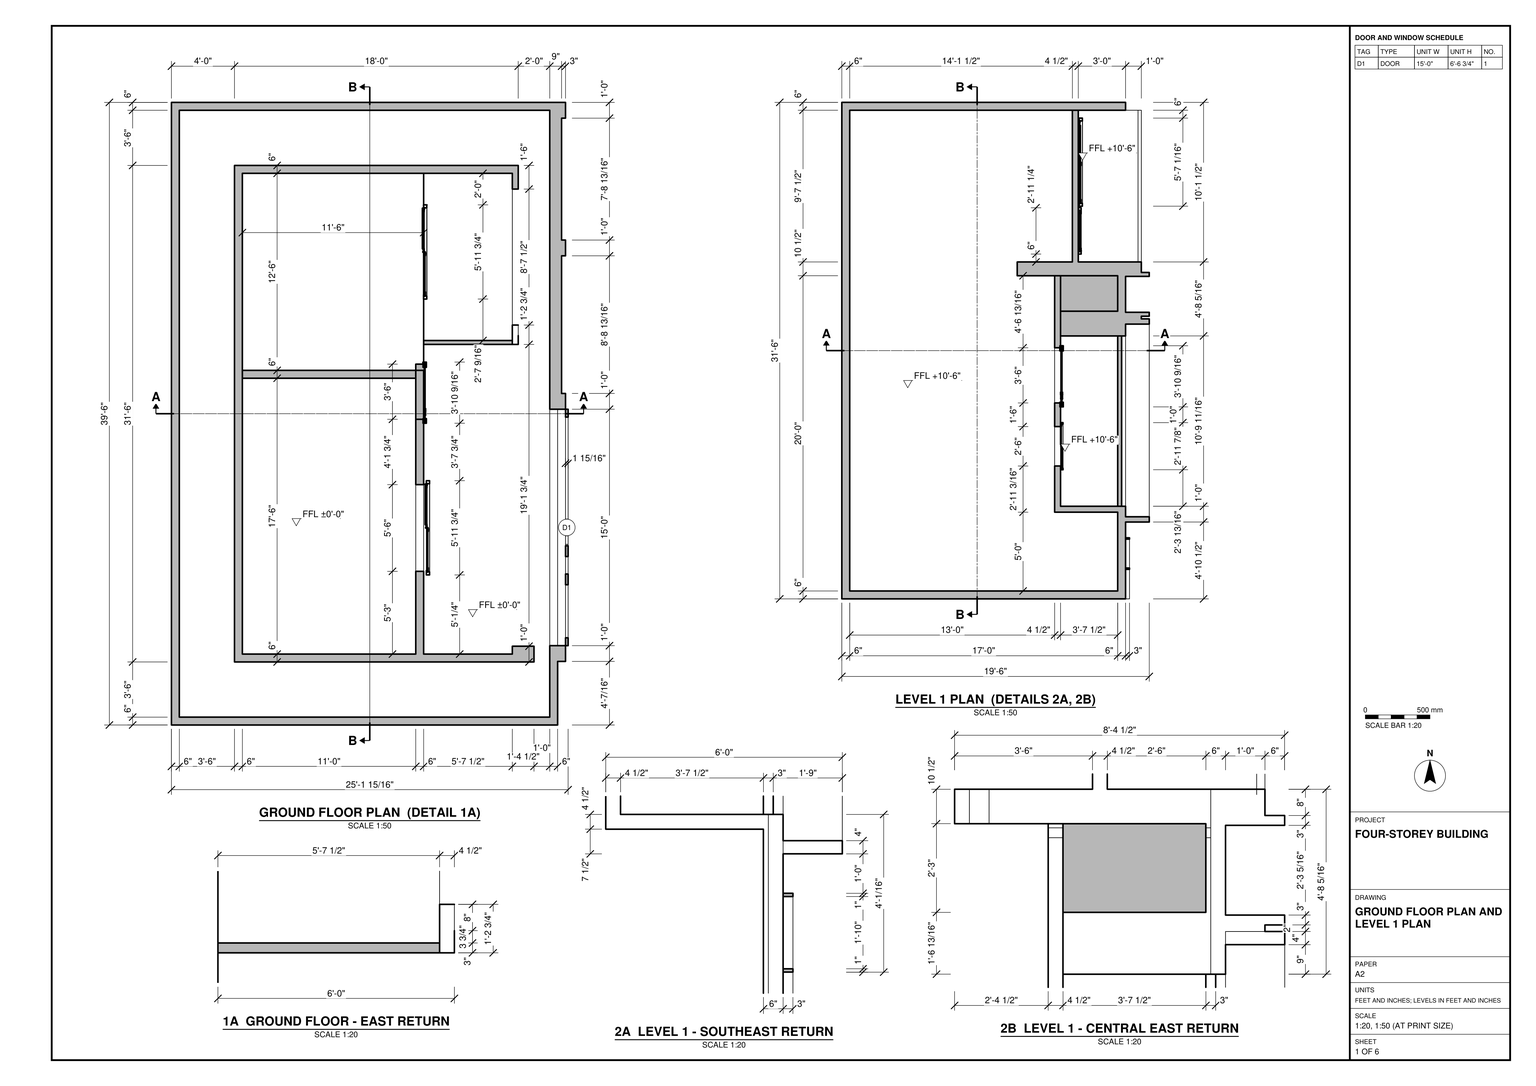
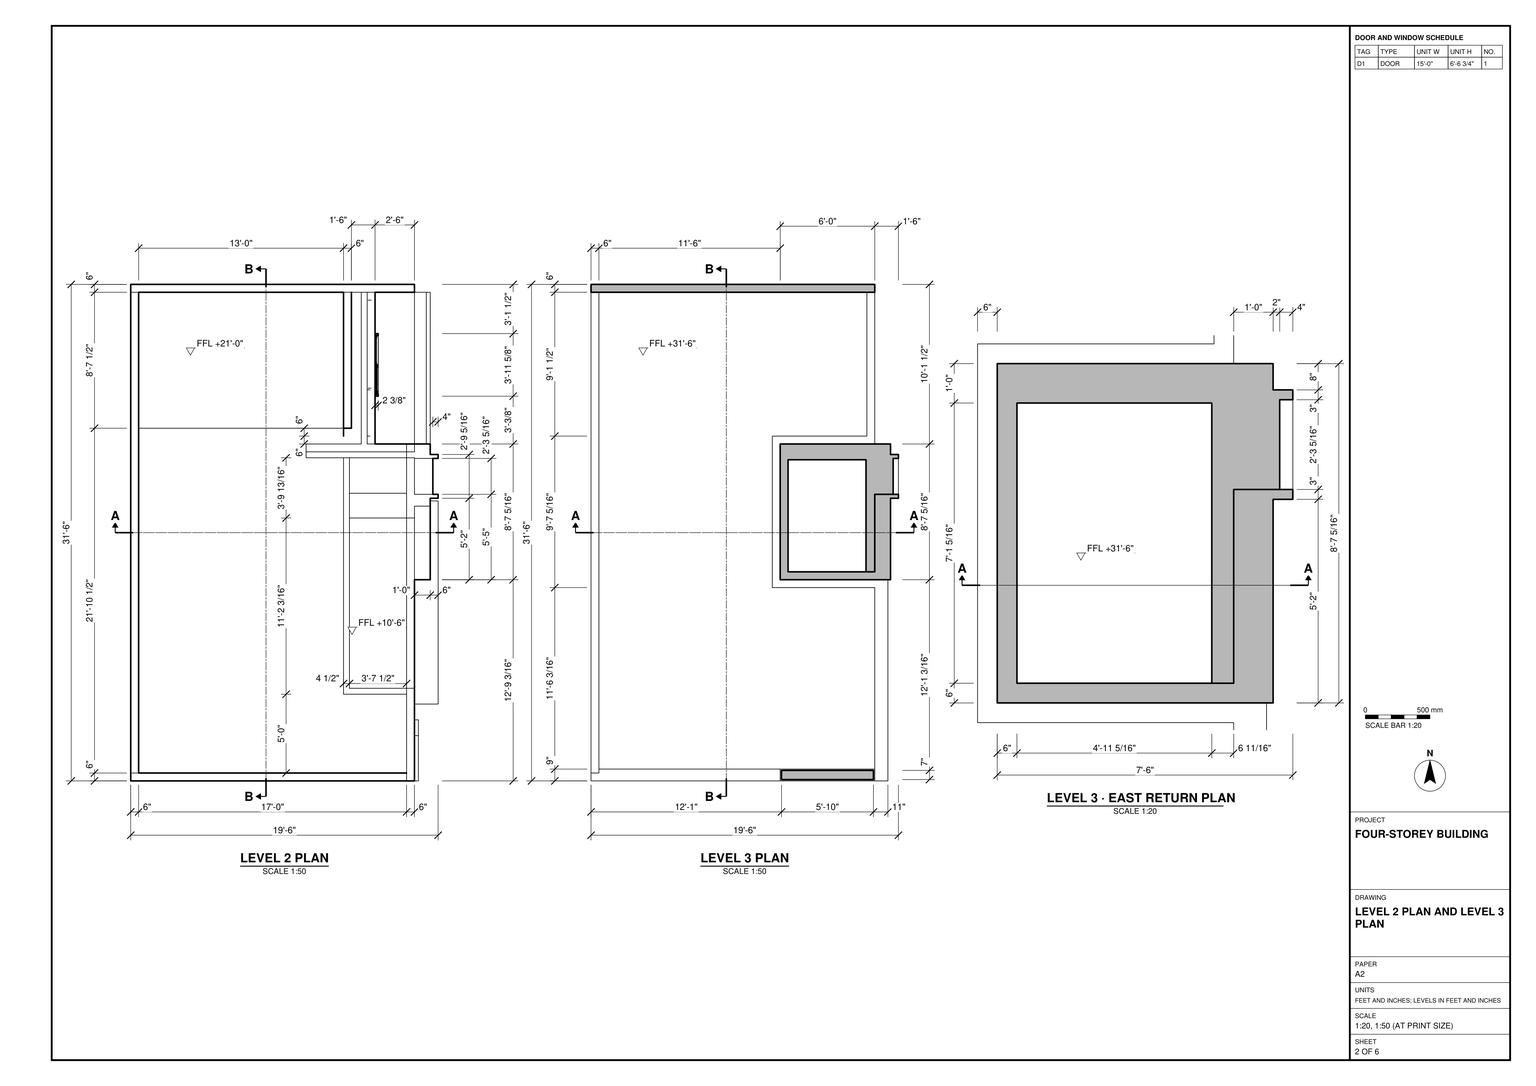
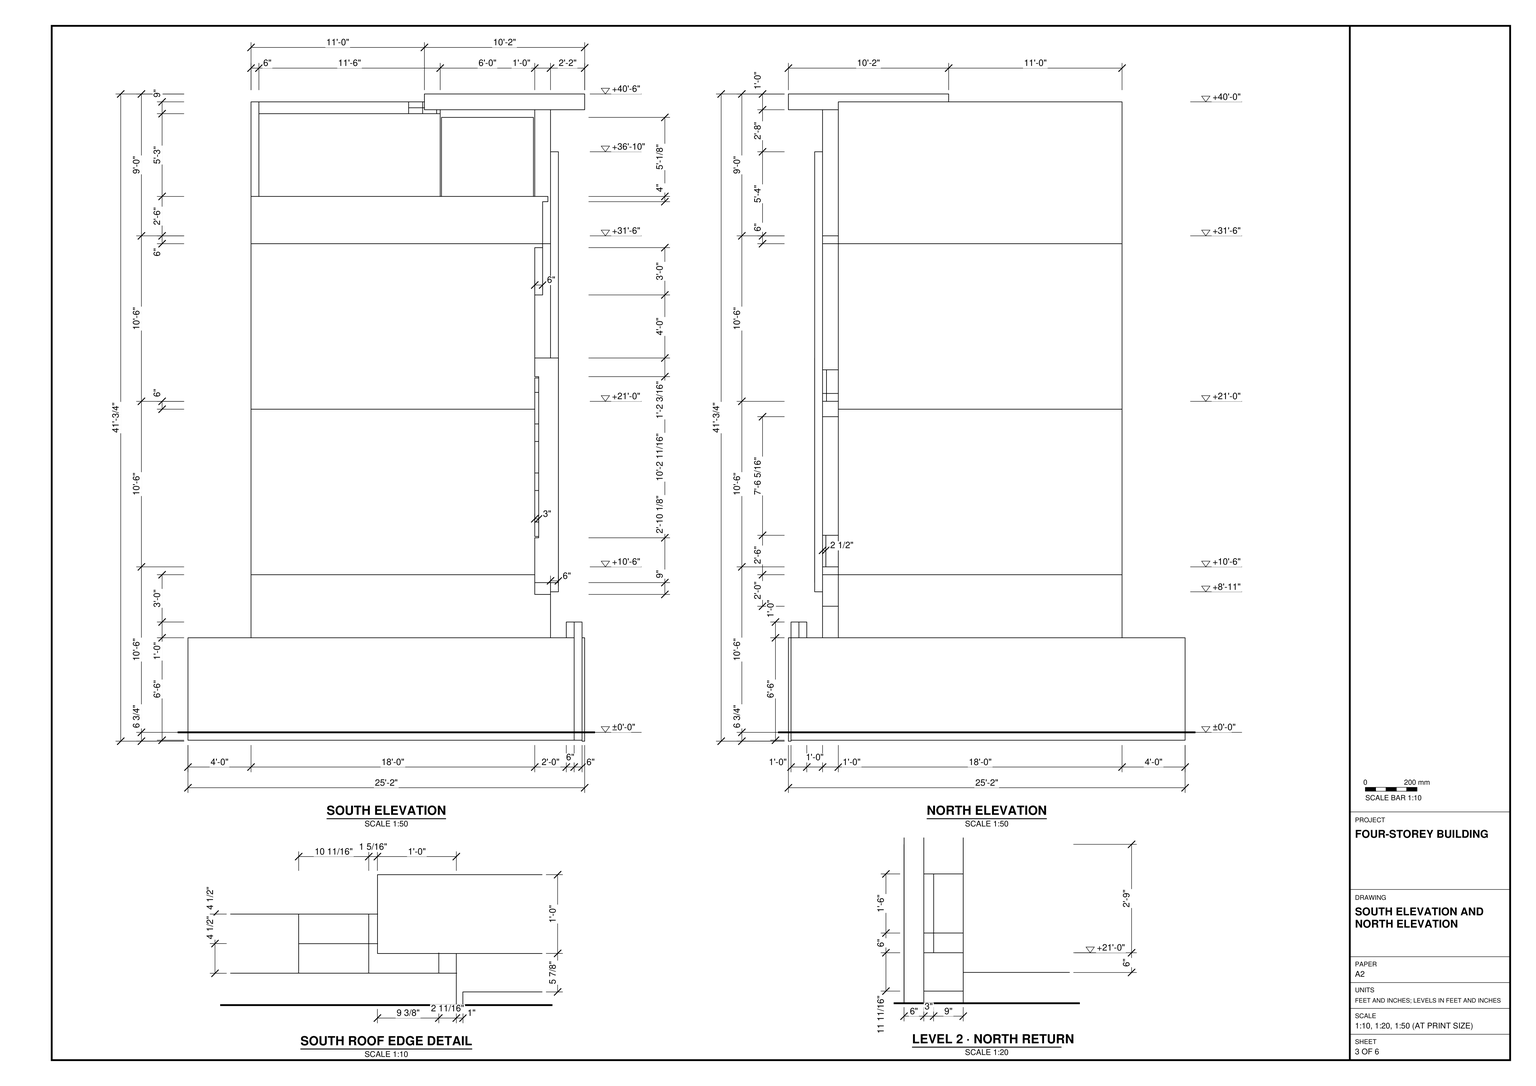
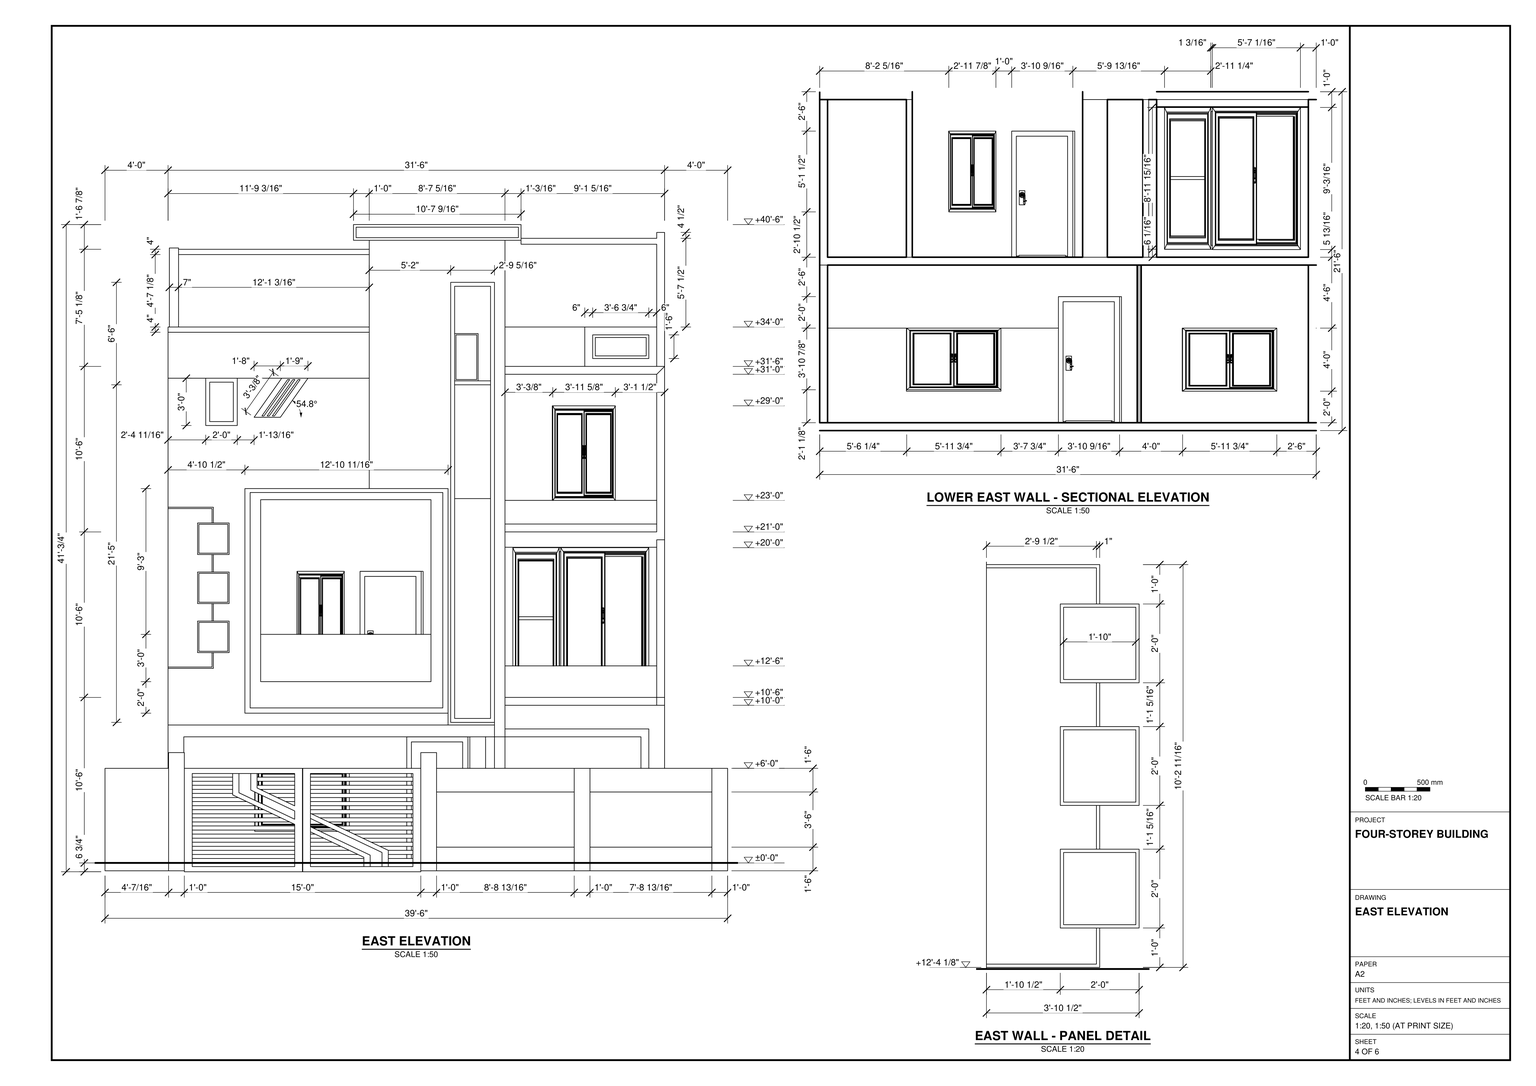
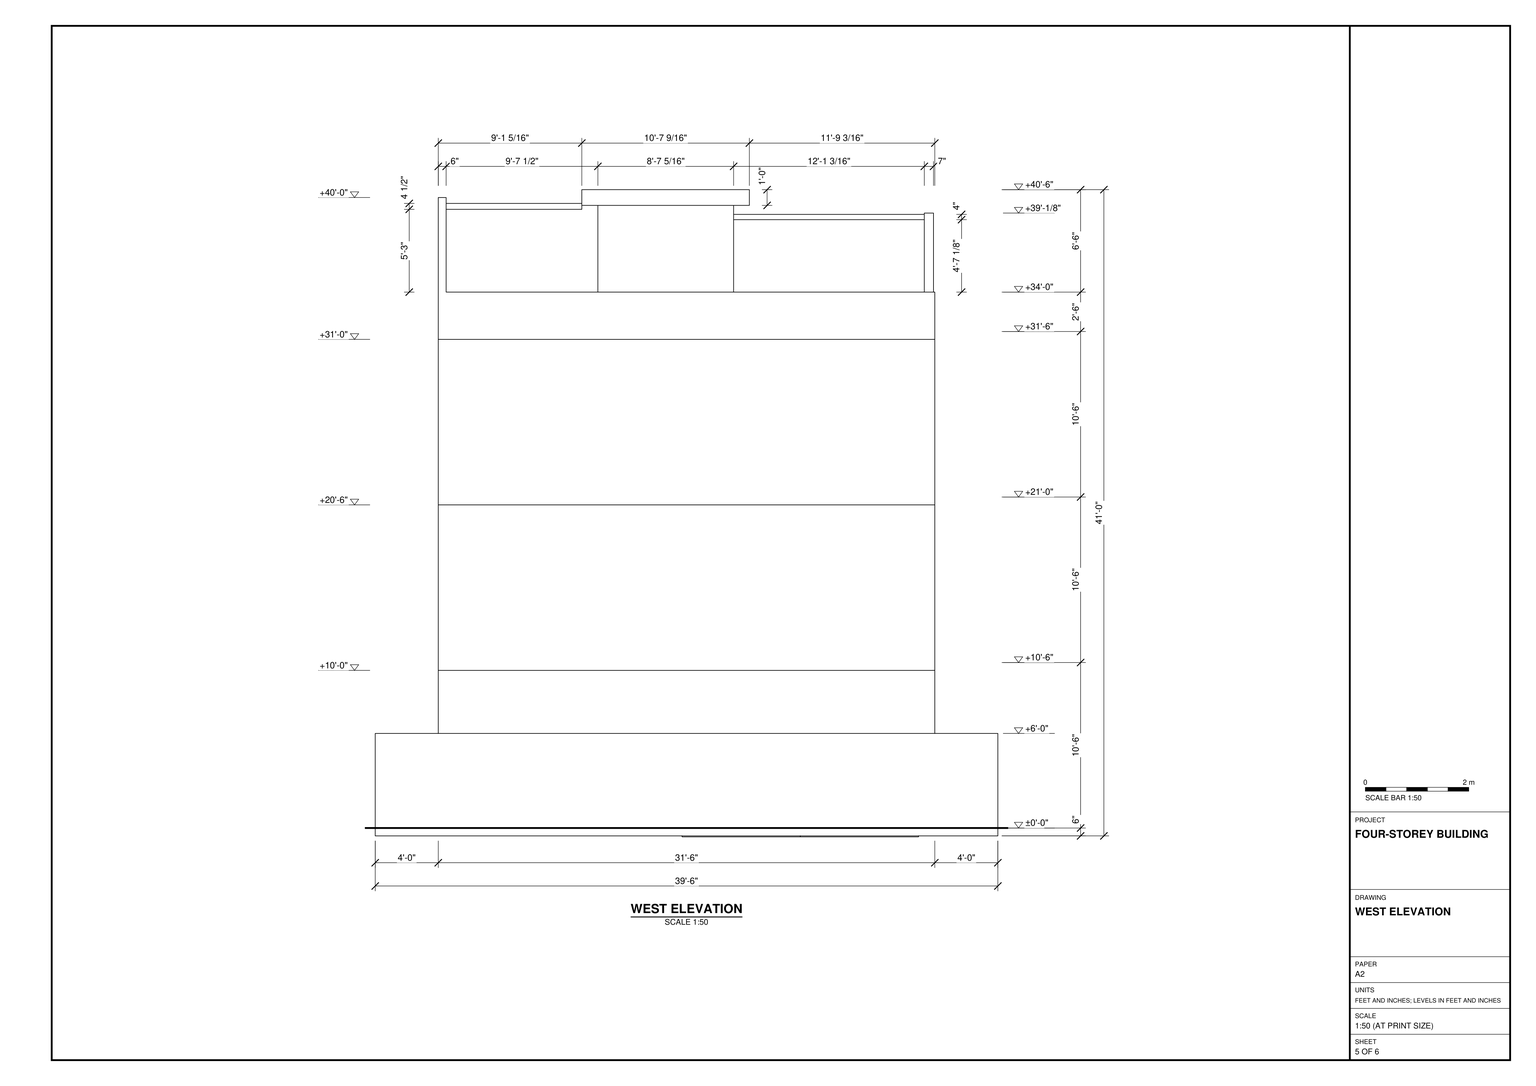
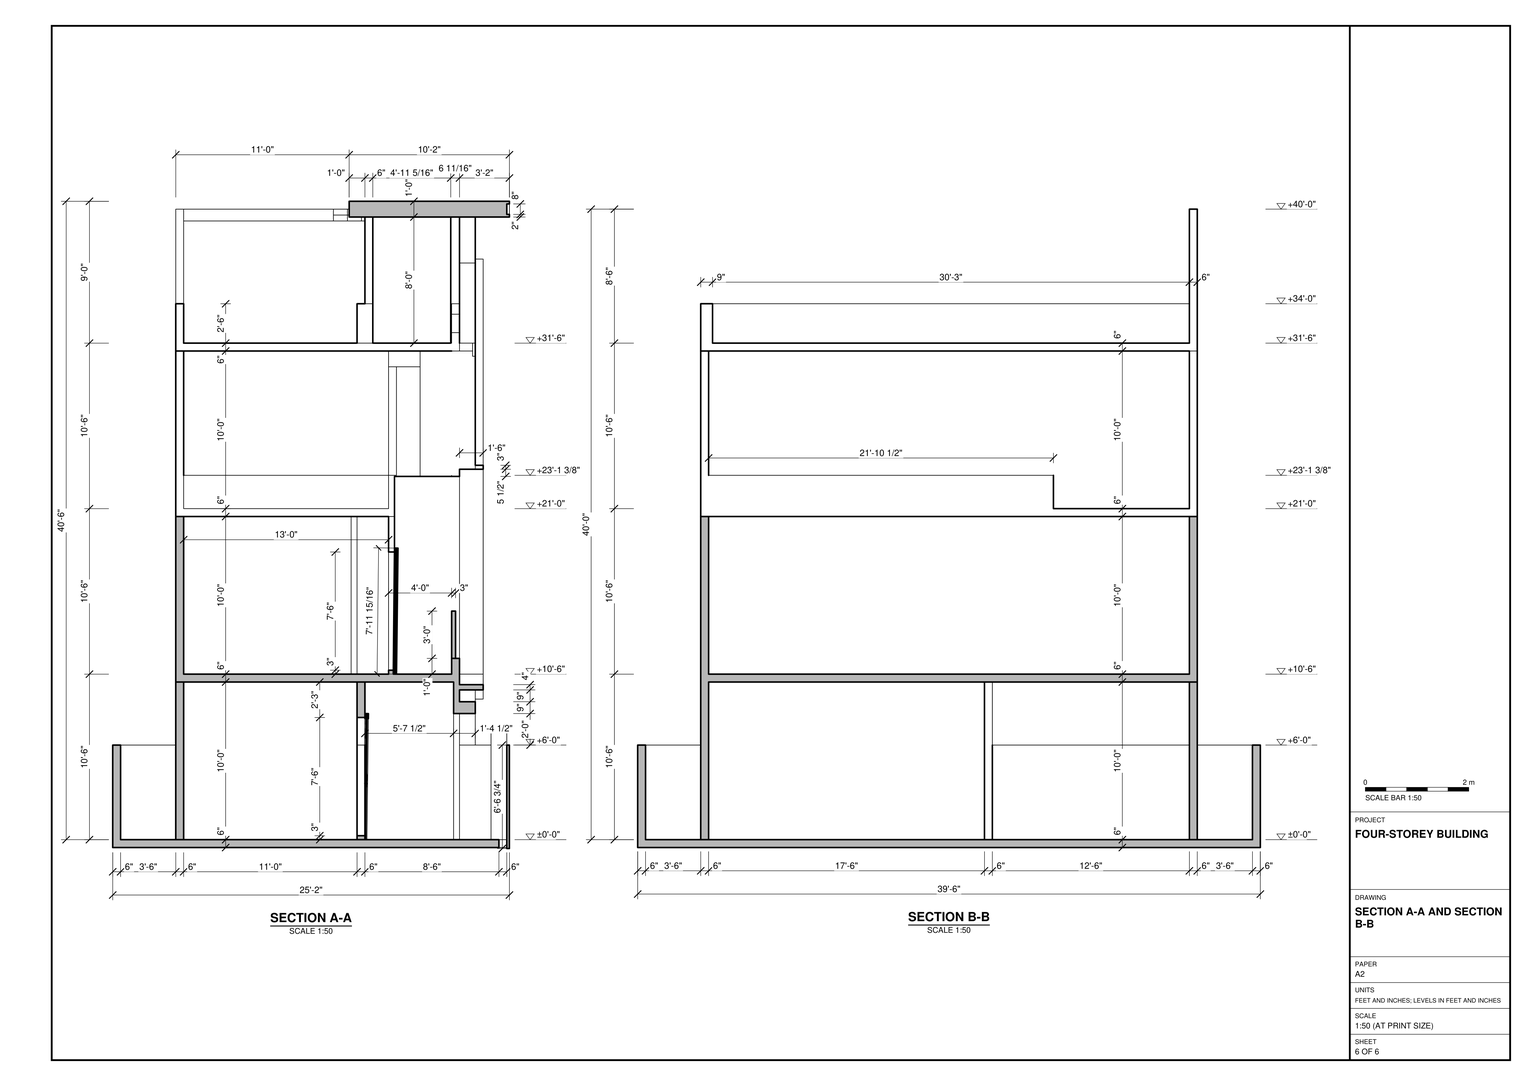
Build the four-storey building in SketchUp from task_files/diagram_01.pdf. Work in feet and inches. The overall model extents are 25'-2" east to west, 39'-6" north to south and 41'-3/4" in height. Set the ground floor at ±0'-0", Level 1 at +10'-6", Level 2 at +21'-0" and Level 3 at +31'-6".

Start with the ground-floor perimeter wall and its wide east entrance gate. Set the building footprint inside the enclosure, leaving the clearances shown in plan. Form the two rooms on the west side with their dividing wall, and follow the plan for the partitions, openings and short wall returns on the east. Use the wall thicknesses shown for each part rather than one thickness throughout.

Build the upper floor slabs to their individual outlines. Use the enlarged east-side details to locate the recesses and projections, retain the opening down to Level 1 beside the Level 2 slab, and form the rectangular return at Level 3. Match the roof overhang and changes in roof-edge height to the elevations. Include stairs, built-in joinery and main furniture only where shown. Decor and loose items may be any suitable library components.

Keep walls, slabs, the roof and each furniture or joinery piece in separate groups or components. Use components for repeated parts. Save one SketchUp model as output_files/four_storey_building_with_gated_ground_floor_enclosure.skp.

# SketchUp Ruby script. Lengths in inches.
U = 1.inch
M = Sketchup.active_model
def pt(a) = Geom::Point3d.new(a.map { |v| v * U })
def face(e, loops, mat)
  f = e.add_face(loops[0].map { |a| pt(a) })
  loops[1..].each { |l| e.add_face(l.map { |a| pt(a) }).erase! }
  f.material = f.back_material = mat if mat
  f
end
# faces: each face lists its corners as indices into pts; further lists are holes
def faces(e, pts, list, mat = nil) = list.each { |f| face(e, (f[0].is_a?(Array) ? f : [f]).map { |l| l.map { |i| pts[i] } }, mat) }
# xy, xz, yz: faces in a plane at the given z, y or x. An outline is a flat list of corners, or four numbers for a rectangle; further outlines are holes
def ring(l) = l.size == 4 ? [[l[0], l[1]], [l[2], l[1]], [l[2], l[3]], [l[0], l[3]]] : l.each_slice(2).to_a
def flat(e, list, mat, &to3) = list.each { |f| face(e, (f[0].is_a?(Array) ? f : [f]).map { |l| ring(l).map { |u, v| to3.(u, v) } }, mat) }
def xy(e, z, list, mat = nil) = flat(e, list, mat) { |x, y| [x, y, z] }
def xz(e, y, list, mat = nil) = flat(e, list, mat) { |x, z| [x, y, z] }
def yz(e, x, list, mat = nil) = flat(e, list, mat) { |y, z| [x, y, z] }
def lines(e, pts, list) = list.each { |a, b| e.add_line(pt(pts[a]), pt(pts[b])) }
# prism: a flat outline (further loops are holes) pulled along v
def prism(e, loops, v, mat = nil)
  f = face(e, loops, mat); d = Geom::Vector3d.new(v.map { |x| x * U })
  f.pushpull(f.normal.samedirection?(d) ? d.length : -d.length)
end
def box(e, o, s, mat = nil) = prism(e, [[o, [o[0] + s[0], o[1], o[2]], [o[0] + s[0], o[1] + s[1], o[2]], [o[0], o[1] + s[1], o[2]]]], [0, 0, s[2]], mat)
def at(x, y, z, deg = 0) = Geom::Transformation.translation(pt([x, y, z])) * Geom::Transformation.rotation(ORIGIN, Z_AXIS, deg.degrees)
def axes(o, x, y, z) = Geom::Transformation.new([*x, 0, *y, 0, *z, 0, *pt(o).to_a, 1])
def part(name) = M.definitions.add(name)
# library, detail: a bought-in or finely detailed component or shape, given as its bounding box
def library(name, o, s) = part(name).tap { |d| box(d.entities, o, s) }
def detail(e, o, s) = box(e.add_group.entities, o, s)
def put(e, d, t, mat = nil) = e.add_instance(d, t).tap { |i| i.material = mat if mat }
def group(e, t, mat = nil) = e.add_group.tap { |g| g.transformation = t; g.material = mat if mat }.entities
root = M.entities
M.materials.add("Brick_20_1K").color = [191, 165, 141]
M.materials.add("Carpet_04_1K").color = [70, 107, 140]
M.materials.add("Carpet_04_1K1").color = [43, 65, 85]
M.materials.add("Denim_03_1K").color = [93, 106, 119]
M.materials.add("Glass_Basic_01").color = [161, 173, 186]
M.materials["Glass_Basic_01"].alpha = 0.25
M.materials.add("I01_Sky_Frost").color = [204, 204, 255]
M.materials.add("[_0053_Ivory_]").color = [200, 200, 200]
c1 = library("porta+4",[0.2,-5.42,1.33],[46.55,4.72,83.21])
c2 = library("Modern+Gate+1",[0,0,0],[118.11,1.97,78.74])
c3 = library("mesh-158",[272.88,-1887.9,-41.96],[1017.57,1401.85,65.81])
c4 = library("mesh-166",[-1553.69,-2604.3125,-42.18],[1702.88,1401.6,88.28])
c5 = part("Group17")
put(c5.entities,c4,at(294.66,859.51,3.5))
c6 = library("mesh-165",[-1596.32,-2661.67,-39.91],[1702.88,1739.15,82.5])
p = [[294,252.41,72],[288,252.41,72],[294,48.41,72],[288,48,72]]
lines(root,p,[[0,1],[2,3]])
put(root,c1,axes([189.24,229.54,-1.54],[0,1,0],[-1,0,0],[0,0,1.15408]))
put(root,c1,axes([211.74,193.97,124.46],[0,1,0],[-1,0,0],[0,0,1.15408]))
g1 = group(root,at(0,0,-6),"[_0053_Ivory_]")
xy(g1,0,[[0,0,0,474,300,474,300,462,294,462,294,369.2,300,369.2,300,357.2,294,357.2,294,252.41,300,252.41,300,240.41,294,240.41,294,60.41,300,60.41,300,48.41,294,48.41,294,0]])
xy(g1,6,[[[6,6,288,468],[54,270,54,420,259.5,420,259.5,304.5,264,304.5,264,289.74,192,289.74,192,270],[54,54,186,264]],[54,54,186,264],[288,60.41,294,240.41],[54,270,192,420],[192,289.74,259.5,292.74],
  [259.5,289.74,264,304.5],[192,292.74,259.5,420]])
xy(g1,9,[[186,232.74,192,270],[186,270,192,274.74]])
xy(g1,18,[[294,252.41,297,357.2],[294,369.2,297,462]])
xy(g1,33,[[186,117,192,183]])
xy(g1,60,[[294,252.41,297,357.2],[294,369.2,297,462]])
xy(g1,75,[[186,117,192,183]])
xy(g1,78,[[0,0,294,0,294,48.41,288,48.41,288,6,6,6,6,468,288,468,288,252.41,294,252.41,294,474,0,474],[294,357.2,300,369.2],[294,462,300,474]])
xy(g1,90,[[288,48.41,300,60.41],[288,240.41,300,252.41]])
xy(g1,99,[[186,232.74,192,274.74]])
xy(g1,102,[[259.5,60,276,289.74],[264,289.74,276,296.5],[259.5,304.5,264,408]])
xy(g1,111,[[264,48,276,261.17]])
xy(g1,113,[[276,263.17,282,296.5]])
xy(g1,116,[[264,266.17,282,293.5]])
xy(g1,120,[[264,106.5,282.03,118.5],[264,118.5,282.03,261.17]])
xy(g1,124,[[264,110.5,282.03,257.17]])
xy(g1,126,[[48,48,54,426],[54,54,186,264],[186,54,192,270],[192,54,259.5,289.74],[54,264,186,270],
  [54,270,186,420],[186,270,192,420],[192,289.74,259.5,292.74],[192,292.74,259.5,420],[264,304.5,276,420],
  [54,420,186,426],[186,420,192,426],[192,420,207,426],[207,420,211.5,426],[211.5,420,259.5,426]])
xy(g1,132,[[54,54,258,54,258,114,210,114,210,294,181.5,294,181.5,304.5,223.5,304.5,223.5,420,54,420],[214.5,118.5,258,248.17],[214.5,267,258,294],[228,304.5,273.48,420],[273.48,304.5,276,420]])
xy(g1,135,[[210,197.17,214.5,239.17]])
xy(g1,144,[[258,118.5,261,248.17],[261,118.5,264,248.17]])
xy(g1,154.12,[[264,48,267,82.49]])
xy(g1,155.12,[[264,48,267,81.49]])
xy(g1,156,[[273.48,304.5,276,420]])
xy(g1,166.12,[[264,70.49,267,81.49],[264,81.49,267,82.49],[264,82.49,267,94.49]])
xy(g1,167.12,[[264,71.49,267,93.49]])
xy(g1,171,[[210,149.17,214.5,179.17]])
xy(g1,180,[[258,118.5,261,248.17]])
xy(g1,189.12,[[264,71.49,267,93.49]])
xy(g1,190.12,[[264,70.49,267,81.49],[264,81.49,267,82.49],[264,82.49,267,94.49]])
xy(g1,203.45,[[264,70.49,267,81.49],[264,81.49,267,82.49],[264,82.49,267,94.49]])
xy(g1,204.45,[[264,71.49,267,93.49]])
xy(g1,225,[[210,149.17,214.5,179.17],[210,197.17,214.5,239.17]])
xy(g1,226.45,[[264,71.49,267,93.49]])
xy(g1,227.45,[[264,70.49,267,81.49],[264,81.49,267,82.49],[264,82.49,267,94.49]])
xy(g1,240.79,[[264,70.49,267,81.49],[264,81.49,267,82.49],[264,82.49,267,94.49]])
xy(g1,241.79,[[264,71.49,267,93.49]])
xy(g1,246.31,[[228,304.5,264,420]])
xy(g1,252,[[48,48,258,54],[48,54,54,420],[54,54,54,420,223.5,420,223.5,304.5,181.5,304.5,181.5,294,210,294,210,114,258,114,258,54],[214.5,267,258,294],[181.5,298.5,181.5,304.5,223.5,304.5,223.5,420,228,420,228,304.5,264,304.5,264,298.5],
  [48,420,264,426]])
xy(g1,258,[[234,304.5,264,420],[264,304.5,273,420],[54,316.5,210,420]])
xy(g1,258,[[273,304.5,276,420]],"Carpet_04_1K")
xy(g1,263.79,[[264,71.49,267,93.49]])
xy(g1,264.79,[[264,70.49,267,81.49],[264,81.49,267,82.49],[264,82.49,267,94.49]])
xy(g1,275.79,[[264,48,267,81.49]])
xy(g1,276.79,[[264,48,267,82.49]])
xy(g1,282,[[273,304.5,276,420]])
xy(g1,282.53,[[214.5,118.5,264,248.17]],"[_0053_Ivory_]")
xy(g1,283.37,[[264,266.17,278,293.5]])
xy(g1,288,[[264,110.5,282.03,257.17]])
xy(g1,291,[[264,106.5,282.03,106.5,282.03,261.17,276,261.17,276,201.17,264,201.17]])
xy(g1,339,[[264,76.69,270,100.69]])
xy(g1,342,[[264,79.69,270,97.69]])
xy(g1,345.27,[[264,113.51,270,133.51]])
xy(g1,346.27,[[268,119.44,270,120.99],[268,123.44,270,124.99],[268,127.44,270,128.99]])
xy(g1,370,[[278,266.17,282,293.5]])
xy(g1,372,[[264,79.69,270,97.69]])
xy(g1,373,[[278,266.17,282,293.5]])
xy(g1,374,[[268,139.02,270,140.57],[268,143.02,270,144.57],[268,147.02,270,148.57],[273.97,267.17,278,283.04]])
xy(g1,375,[[264,48,270,76.69],[264,100.69,270,134.5],[264,154.5,270,201.17]])
xy(g1,378,[[48,48,54,420],[54,48,258,54],[54,54,54,420,210,420,210,310.5,234,310.5,234,304.5,258,304.5,258,54],[234,304.5,264,420],[210,310.5,234,316.5]])
xy(g1,384,[[54,57,264,57,264,195.17,186,195.17,186,310.5,258,310.5,258,420,54,420],[198,207.17,257.33,292.5]])
xy(g1,392,[[258,373.25,264,412]])
xy(g1,406,[[258,373.25,264,412]])
xy(g1,408,[[273.97,267.17,278,283.04]])
xy(g1,410,[[270,48,274,54],[270,54,274,201.17]],"[_0053_Ivory_]")
xy(g1,414,[[48,48,192,48,192,57,54,57,54,54,48,54],[264,48,274,48,274,201.17,192,201.17,192,304.5,264,304.5,264,420,258,420,258,310.5,186,310.5,186,195.17,264,195.17],[[192,48,264,57],[193,49,263,56]],[48,54,54,420]])
xy(g1,445,[[264,266.17,278,292.5],[278,266.17,282,292.5],[278,292.5,282,293.5]])
xy(g1,448,[[276,263.17,282,296.5]])
xy(g1,469.15,[[[194,56,262,201.17],[209,71,247,76.02],[209,82.02,247,87.03],[209,93.03,247,98.05],[209,104.05,247,109.0625],[209,115.0625,247,120.08],[209,137.09,247,142.11],[209,148.11,247,153.125],[209,159.125,247,164.14],[209,170.14,247,175.15],[209,181.15,247,186.17],[209,126.08,247,131.09]]])
xy(g1,473.15,[[[194,56,262,201.17],[206,68,250,189.17]],[[206,68,250,79.02],[209,71,247,76.02]],[[206,79.02,250,90.03],[209,82.02,247,87.03]],[[206,90.03,250,101.05],[209,93.03,247,98.05]],[[206,101.05,250,112.0625],[209,104.05,247,109.0625]],
  [[206,112.0625,250,123.08],[209,115.0625,247,120.08]],[[206,123.08,250,134.09],[209,126.08,247,131.09]],[[206,134.09,250,145.11],[209,137.09,247,142.11]],[[206,145.11,250,156.125],[209,148.11,247,153.125]],[[206,156.125,250,167.14],[209,159.125,247,164.14]],
  [[206,167.14,250,178.15],[209,170.14,247,175.15]],[[206,178.15,250,189.17],[209,181.15,247,186.17]]])
xy(g1,474.15,[[193,49,263,56]])
xy(g1,477,[[168,316.72,178.67,420],[189.33,316.72,200,420],[210.67,316.72,221.33,420],[232,316.72,242.67,420],[253.33,316.72,264,420]])
xy(g1,480,[[180,189.17,264,201.17],[264,189.17,276,201.17],[276,189.17,302,207.17],[180,201.17,192,207.17],[192,201.17,276,207.17],
  [180,207.17,192,304.5],[192,207.17,198,304.5],[198,207.17,257.33,292.5],[257.33,207.17,264,304.5],[264,207.17,276,304.5],
  [276,207.17,302,316.72],[198,292.5,257.33,304.5],[180,304.5,198,316.72],[198,304.5,257.33,316.72],[257.33,304.5,264,316.72],
  [264,304.5,276,316.72]])
xy(g1,481.5,[[168,316.72,178.67,420],[189.33,316.72,200,420],[210.67,316.72,221.33,420],[232,316.72,242.67,420],[253.33,316.72,264,420]])
xy(g1,482,[[300,191.17,302,207.17],[300,207.17,302,314.72]])
xy(g1,486,[[48,420,264,426]])
xy(g1,490,[[300,191.17,302,314.72]])
xy(g1,492,[[180,189.17,302,316.72]])
xz(g1,0,[[0,0,294,78]])
xz(g1,6,[[6,6,48,78],[48,6,240,78],[240,6,246,78],[246,6,288,78]])
xz(g1,48,[[48,6,276,6,276,111,264,111,264,126,48,126],[48,126,264,126,264,154.12,267,154.12,267,155.12,264,155.12,264,252,48,252],[48,252,264,252,264,275.79,267,275.79,267,276.79,264,276.79,264,375,270,375,270,378,48,378],[48,378,270,378,270,410,274,410,274,414,48,414]])
xz(g1,48.41,[[294,0,300,6],[294,6,300,90],[288,78,294,90]])
xz(g1,49,[[193,414,263,474.15]])
xz(g1,54,[[54,6,186,126],[192,6,259.5,78],[192,78,259.5,126],[54,132,258,252],[54,283.37,258,378]])
xz(g1,56,[[193,414,263,468.15],[[193,468.15,263,474.15],[194,469.15,262,473.15]]])
xz(g1,57,[[54,384,264,414]])
xz(g1,60,[[259.5,6,264,78],[264,6,264,78,259.5,78,259.5,102,276,102,276,6]])
xz(g1,60.41,[[294,0,300,6],[288,6,300,90]])
xz(g1,70.49,[[264,166.12,267,190.12],[264,203.45,267,227.45],[264,240.79,267,264.79]])
xz(g1,71,[[209,469.15,247,473.15]])
xz(g1,71.49,[[264,167.12,267,189.12],[264,204.45,267,226.45],[264,241.79,267,263.79]])
xz(g1,76.02,[[209,469.15,247,473.15]])
xz(g1,76.69,[[264,339,270,375]])
xz(g1,79.69,[[264,342,270,372]])
xz(g1,81.49,[[264,155.12,267,166.12],[264,190.12,267,203.45],[264,227.45,267,240.79],[264,264.79,267,275.79]])
xz(g1,82.02,[[209,469.15,247,473.15]])
xz(g1,82.49,[[264,154.12,267,166.12],[264,190.12,267,203.45],[264,227.45,267,240.79],[264,264.79,267,276.79]])
xz(g1,87.03,[[209,469.15,247,473.15]])
xz(g1,93.03,[[209,469.15,247,473.15]])
xz(g1,93.49,[[264,167.12,267,189.12],[264,204.45,267,226.45],[264,241.79,267,263.79]])
xz(g1,94.49,[[264,166.12,267,190.12],[264,203.45,267,227.45],[264,240.79,267,264.79]])
xz(g1,97.69,[[264,342,270,372]])
xz(g1,98.05,[[209,469.15,247,473.15]])
xz(g1,100.69,[[264,339,270,375]])
xz(g1,104.05,[[209,469.15,247,473.15]])
xz(g1,106.5,[[264,120,282.03,291]])
xz(g1,109.0625,[[209,469.15,247,473.15]])
xz(g1,110.5,[[264,124,282.03,288]])
xz(g1,114,[[210,132,258,252]])
xz(g1,115.0625,[[209,469.15,247,473.15]])
xz(g1,117,[[186,33,192,75]])
xz(g1,118.5,[[258,144,261,180]])
xz(g1,118.5,[[214.5,132,214.5,282.53,264,282.53,264,144,261,144,261,180,258,180,258,132]],"[_0053_Ivory_]")
xz(g1,120.08,[[209,469.15,247,473.15]])
xz(g1,126.08,[[209,469.15,247,473.15]])
xz(g1,131.09,[[209,469.15,247,473.15]])
xz(g1,137.09,[[209,469.15,247,473.15]])
xz(g1,142.11,[[209,469.15,247,473.15]])
xz(g1,148.11,[[209,469.15,247,473.15]])
xz(g1,149.17,[[210,171,214.5,225]])
xz(g1,153.125,[[209,469.15,247,473.15]])
xz(g1,159.125,[[209,469.15,247,473.15]])
xz(g1,164.14,[[209,469.15,247,473.15]])
xz(g1,170.14,[[209,469.15,247,473.15]])
xz(g1,175.15,[[209,469.15,247,473.15]])
xz(g1,179.17,[[210,171,214.5,225]])
xz(g1,181.15,[[209,469.15,247,473.15]])
xz(g1,183,[[186,33,192,75]])
xz(g1,186.17,[[209,469.15,247,473.15]])
xz(g1,189.17,[[180,480,302,492]])
xz(g1,191.17,[[300,482,302,490]])
xz(g1,195.17,[[186,384,264,414]])
xz(g1,197.17,[[210,135,214.5,225]])
xz(g1,201.17,[[264,291,276,291,276,378,270,378,270,375,264,375],[270,378,276,378,276,480,264,480,264,414,274,414,274,410,270,410],[[192,414,264,480],[194,469.15,262,473.15]]])
xz(g1,207.17,[[198,384,257.33,480],[257.33,384,264,480]])
xz(g1,232.74,[[186,9,192,99]])
xz(g1,239.17,[[210,135,214.5,225]])
xz(g1,240.41,[[294,0,300,6],[288,6,300,90]])
xz(g1,248.17,[[258,144,261,180]])
xz(g1,248.17,[[214.5,132,258,132,258,180,261,180,261,144,264,144,264,282.53,214.5,282.53]],"[_0053_Ivory_]")
xz(g1,252.41,[[294,0,300,6],[294,6,294,18,297,18,297,60,294,60,294,90,300,90,300,6],[288,78,294,90]])
xz(g1,257.17,[[264,124,282.03,132],[264,132,282.03,288]])
xz(g1,261.17,[[264,111,276,120],[276,120,282.03,291]])
xz(g1,263.17,[[276,113,282,120],[276,120,282,448]])
xz(g1,264,[[54,6,186,126]])
xz(g1,266.17,[[264,116,282,283.37],[278,283.37,282,370],[278,373,282,445],[264,384,278,445]])
xz(g1,267,[[214.5,132,258,252]])
xz(g1,267.17,[[273.97,374,278,408]])
xz(g1,270,[[54,6,192,78]])
xz(g1,274.74,[[186,9,192,99]])
xz(g1,283.04,[[273.97,374,278,408]])
xz(g1,289.74,[[192,6,259.5,126],[259.5,6,264,102]])
xz(g1,292.5,[[198,384,257.33,480]])
xz(g1,292.74,[[192,6,259.5,126]])
xz(g1,293.5,[[264,116,282,126],[264,126,282,132],[264,132,282,283.37],[278,283.37,282,370],[278,373,282,406],
  [278,406,282,409],[278,409,282,445]])
xz(g1,294,[[181.5,132,186,252],[186,132,210,252],[210,132,214.5,252],[214.5,132,258,252]])
xz(g1,296.5,[[264,78,276,102],[276,113,282,448]])
xz(g1,304.5,[[259.5,6,264,78],[259.5,78,276,102],[264,102,276,126],[181.5,132,223.5,252],[228,132,228,246.31,276,246.31,276,156,273.48,156,273.48,132],
  [273.48,132,276,156],[228,246.31,264,252],[234,258,234,378,276,378,276,282,273,282,273,258],[273,258,276,282],[264,384,264,414,192,414,192,480,276,480,276,384]])
xz(g1,304.5,[[264,246.31,276,258],[264,378,276,384]],"Carpet_04_1K")
xz(g1,310.5,[[186,384,258,414]])
xz(g1,314.72,[[300,482,302,490]])
xz(g1,316.5,[[54,258,210,283.37],[210,283.37,216,366]])
xz(g1,316.72,[[168,477,178.67,481.5],[189.33,477,200,480],[210.67,477,221.33,480],[232,477,242.67,480],[253.33,477,264,480],
  [180,480,180,492,302,492,302,480,264,480,264,481.5,253.33,481.5,253.33,480,242.67,480,242.67,481.5,232,481.5,232,480,221.33,480,221.33,481.5,210.67,481.5,210.67,480,200,480,200,481.5,189.33,481.5,189.33,480],[189.33,480,200,481.5],[210.67,480,221.33,481.5],[232,480,242.67,481.5],[253.33,480,264,481.5]])
xz(g1,357.2,[[294,0,300,0,300,78,294,78,294,60,297,60,297,18,294,18]])
xz(g1,369.2,[[294,0,294,18,297,18,297,60,294,60,294,78,300,78,300,0]])
xz(g1,373.25,[[258,392,264,406]])
xz(g1,408,[[259.5,6,264,102]])
xz(g1,412,[[258,392,264,406]])
xz(g1,420,[[54,6,192,78],[192,6,259.5,126],[54,78,192,126],[54,132,223.5,252],[223.5,132,228,252],
  [228,132,264,246.31],[264,132,273.48,156],[273.48,132,276,156],[228,246.31,264,252],[54,258,210,378],
  [234,258,264,378],[264,258,273,264],[264,264,273,282],[54,384,258,384,258,414,264,414,264,477,54,477],[48,414,54,486],
  [54,477,168,486],[178.67,477,189.33,481.5],[200,477,210.67,481.5],[221.33,477,232,481.5],[242.67,477,253.33,481.5],
  [168,481.5,178.67,486],[178.67,481.5,189.33,486],[189.33,481.5,200,486],[200,481.5,210.67,486],[210.67,481.5,221.33,486],
  [221.33,481.5,232,486],[232,481.5,242.67,486],[242.67,481.5,253.33,486],[253.33,481.5,264,486]])
xz(g1,420,[[264,126,276,132],[273,258,276,264],[273,264,276,282]],"Carpet_04_1K")
xz(g1,426,[[48,6,264,126],[48,126,264,252],[48,252,264,378],[48,378,264,486]])
xz(g1,462,[[294,0,300,0,300,78,294,78,294,60,297,60,297,18,294,18]])
xz(g1,468,[[6,6,48,78],[48,6,288,78]])
xz(g1,474,[[0,0,300,78]])
yz(g1,0,[[0,0,474,78]])
yz(g1,6,[[6,6,54,78],[54,6,264,78],[264,6,420,78],[420,6,426,78],[426,6,468,78]])
yz(g1,48,[[48,6,426,126],[48,126,426,252],[48,252,426,378],[48,378,48,414,420,414,420,486,426,486,426,378]])
yz(g1,54,[[54,6,264,126],[264,6,270,126],[270,6,420,78],[270,78,420,126],[54,132,420,252],
  [316.5,258,420,258,420,378,54,378,54,283.37,316.5,283.37],[57,384,420,414]])
yz(g1,168,[[316.72,477,420,481.5]])
yz(g1,178.67,[[316.72,477,420,481.5]])
yz(g1,180,[[189.17,480,316.72,492]])
yz(g1,181.5,[[294,132,298.5,252],[298.5,132,304.5,252]])
yz(g1,186,[[[54,6,54,126,264,126,264,99,232.74,99,232.74,9,264,9,264,6],[117,33,183,75]],[232.74,9,264,99],[264,9,274.74,99],[195.17,384,310.5,414]])
yz(g1,189.33,[[316.72,477,420,481.5]])
yz(g1,192,[[229.74,6,270,6,270,9,232.74,9,232.74,78,229.74,78],[270,6,277.74,6,277.74,102,229.74,102,229.74,78,232.74,78,232.74,99,274.74,99,274.74,9,270,9],[289.74,6,292.74,126],[232.74,9,270,78],[[114,30,186,78],[117,33,183,75]],
  [[324,30,396,78],[327,33,393,75]],[327,33,393,75],[201.17,414,304.5,480]])
yz(g1,192,[[277.74,6,289.74,6,289.74,126,54,126,54,78,229.74,78,229.74,102,277.74,102],[54,6,229.74,6,229.74,78,186,78,186,30,114,30,114,78,54,78],[[292.74,6,420,126],[324,30,396,78]]],"Brick_20_1K")
yz(g1,193,[[49,414,56,474.15]])
yz(g1,194,[[56,469.15,201.17,473.15]])
yz(g1,198,[[207.17,384,292.5,480]])
yz(g1,200,[[316.72,477,420,481.5]])
yz(g1,209,[[71,469.15,76.02,473.15],[82.02,469.15,87.03,473.15],[93.03,469.15,98.05,473.15],[104.05,469.15,109.0625,473.15],[115.0625,469.15,120.08,473.15],
  [126.08,469.15,131.09,473.15],[137.09,469.15,142.11,473.15],[148.11,469.15,153.125,473.15],[159.125,469.15,164.14,473.15],[170.14,469.15,175.15,473.15],
  [181.15,469.15,186.17,473.15]])
yz(g1,210,[[[114,132,294,252],[197.17,135,239.17,225],[149.17,171,179.17,225]],[316.5,258,420,378],[310.5,283.37,316.5,378]])
yz(g1,210.67,[[316.72,477,420,481.5]])
yz(g1,214.5,[[[194.17,132,242.17,228],[197.17,135,239.17,225]],[248.17,132,267,252],[267,132,294,252],[[146.17,168,182.17,228],[149.17,171,179.17,225]]])
yz(g1,214.5,[[[118.5,132,194.17,132,194.17,228,242.17,228,242.17,132,248.17,132,248.17,282.53,118.5,282.53],[146.17,168,182.17,228]]],"[_0053_Ivory_]")
yz(g1,216,[[316.5,283.37,420,366]])
yz(g1,221.33,[[316.72,477,420,481.5]])
yz(g1,223.5,[[304.5,132,420,252]])
yz(g1,228,[[[310.5,138,414,246],[313.5,141,313.5,243,344,243,344,141,346,141,346,243,378.5,243,378.5,141,380.5,141,380.5,243,411,243,411,141]],[313.5,141,344,243],[346,141,378.5,243],[380.5,141,411,243],[304.5,246.31,420,252]])
yz(g1,228,[[[304.5,132,420,246.31],[310.5,138,414,246]]],"Denim_03_1K")
yz(g1,232,[[316.72,477,420,481.5]])
yz(g1,234,[[[340.5,282,388.5,354],[343.5,285,385.5,351]],[343.5,285,385.5,351]])
yz(g1,234,[[[304.5,258,420,378],[340.5,282,388.5,354]]],"Denim_03_1K")
yz(g1,242.67,[[316.72,477,420,481.5]])
yz(g1,247,[[71,469.15,76.02,473.15],[82.02,469.15,87.03,473.15],[93.03,469.15,98.05,473.15],[104.05,469.15,109.0625,473.15],[115.0625,469.15,120.08,473.15],
  [126.08,469.15,131.09,473.15],[137.09,469.15,142.11,473.15],[148.11,469.15,153.125,473.15],[159.125,469.15,164.14,473.15],[170.14,469.15,175.15,473.15],
  [181.15,469.15,186.17,473.15]])
yz(g1,253.33,[[316.72,477,420,481.5]])
yz(g1,257.33,[[207.17,384,292.5,480]])
yz(g1,258,[[54,132,114,252],[267,132,294,252],[[310.5,384,420,414],[373.25,392,412,406]]])
yz(g1,258,[[118.5,132,229.62,144],[229.62,132,248.17,144],[118.5,144,248.17,180]],"Glass_Basic_01")
yz(g1,259.5,[[54,6,60,78],[289.74,6,292.74,126],[292.74,6,292.74,126,420,126,420,78,408,78,408,102,304.5,102,304.5,6],[408,6,420,78],[54,78,54,126,289.74,126,289.74,102,60,102,60,78]])
yz(g1,261,[[118.5,144,248.17,180]],"Glass_Basic_01")
yz(g1,262,[[56,469.15,201.17,473.15]])
yz(g1,263,[[49,414,56,474.15]])
yz(g1,264,[[289.74,6,296.5,78],[408,6,414,6,414,108,304.5,108,304.5,102,408,102],[289.74,78,296.5,102],[[110.5,124,257.17,288],[118.5,144,248.17,282.53]],[48,155.12,81.49,155.12,81.49,166.12,70.49,166.12,70.49,190.12,81.49,190.12,81.49,203.45,70.49,203.45,70.49,227.45,81.49,227.45,81.49,240.79,70.49,240.79,70.49,264.79,81.49,264.79,81.49,275.79,48,275.79],
  [70.49,166.12,81.49,166.12,81.49,167.12,71.49,167.12,71.49,189.12,81.49,189.12,81.49,190.12,70.49,190.12],[81.49,166.12,82.49,167.12],[82.49,166.12,94.49,166.12,94.49,190.12,82.49,190.12,82.49,189.12,93.49,189.12,93.49,167.12,82.49,167.12],[71.49,167.12,93.49,189.12],[81.49,189.12,82.49,190.12],
  [70.49,203.45,81.49,203.45,81.49,204.45,71.49,204.45,71.49,226.45,81.49,226.45,81.49,227.45,70.49,227.45],[81.49,203.45,82.49,204.45],[82.49,203.45,94.49,203.45,94.49,227.45,82.49,227.45,82.49,226.45,93.49,226.45,93.49,204.45,82.49,204.45],[71.49,204.45,93.49,226.45],[81.49,226.45,82.49,227.45],
  [70.49,240.79,81.49,240.79,81.49,241.79,71.49,241.79,71.49,263.79,81.49,263.79,81.49,264.79,70.49,264.79],[81.49,240.79,82.49,241.79],[82.49,240.79,94.49,240.79,94.49,264.79,82.49,264.79,82.49,263.79,93.49,263.79,93.49,241.79,82.49,241.79],[71.49,241.79,93.49,263.79],[81.49,263.79,82.49,264.79],
  [79.69,342,97.69,372],[57,384,195.17,414],[207.17,384,207.17,480,292.5,480,292.5,445,266.17,445,266.17,384],[304.5,384,365.25,414],[420,384,426,384,426,486,420,486,420,481.5,316.72,481.5,316.72,477,420,477],
  [[365.25,384,420,414],[371.25,390,414,408]],[[371.25,390,414,408],[373.25,392,412,406]]])
yz(g1,264,[[266.17,116,293.5,283.37]],"Brick_20_1K")
yz(g1,264,[[414,6,426,6,426,126,304.5,126,304.5,108,414,108],[420,126,426,132],[420,132,426,252],[304.5,246.31,420,246.31,420,252,426,252,426,384,420,378,420,258,304.5,258],[304.5,378,420,378,426,384,304.5,384]],"Carpet_04_1K")
yz(g1,264,[[48,111,261.17,111,261.17,120,106.5,120,106.5,291,201.17,291,201.17,375,154.5,375,133.51,345.27,113.51,345.27,134.5,375,100.69,375,100.69,339,76.69,339,76.69,375,48,375,48,276.79,82.49,276.79,82.49,264.79,94.49,264.79,94.49,240.79,82.49,240.79,82.49,227.45,94.49,227.45,94.49,203.45,82.49,203.45,82.49,190.12,94.49,190.12,94.49,166.12,82.49,166.12,82.49,154.12,48,154.12]],"[_0053_Ivory_]")
yz(g1,267,[[48,154.12,82.49,154.12,82.49,166.12,81.49,166.12,81.49,155.12,48,155.12],[[70.49,166.12,94.49,190.12],[71.49,167.12,93.49,189.12]],[81.49,190.12,82.49,203.45],[[70.49,203.45,94.49,227.45],[71.49,204.45,93.49,226.45]],[81.49,227.45,82.49,240.79],
  [[70.49,240.79,94.49,264.79],[71.49,241.79,93.49,263.79]],[81.49,264.79,82.49,264.79,82.49,276.79,48,276.79,48,275.79,81.49,275.79]])
yz(g1,268,[[119.44,346.27,120.99,346.27,140.57,374,139.02,374],[123.44,346.27,124.99,346.27,144.57,374,143.02,374],[127.44,346.27,128.99,346.27,148.57,374,147.02,374]])
yz(g1,270,[[[76.69,339,100.69,375],[79.69,342,97.69,372]],[[113.51,345.27,133.51,345.27,154.5,375,134.5,375],[127.44,346.27,147.02,374,148.57,374,128.99,346.27],[119.44,346.27,139.02,374,140.57,374,120.99,346.27],[123.44,346.27,143.02,374,144.57,374,124.99,346.27]]])
yz(g1,270,[[48,375,201.17,410]],"[_0053_Ivory_]")
yz(g1,273,[[304.5,258,420,282]],"Glass_Basic_01")
yz(g1,273.48,[[304.5,132,420,156]],"Glass_Basic_01")
yz(g1,273.97,[[267.17,374,283.04,408]],"I01_Sky_Frost")
yz(g1,274,[[48,410,201.17,414]],"[_0053_Ivory_]")
yz(g1,276,[[48,6,60,6,60,102,296.5,102,296.5,111,48,111],[304.5,126,420,132]])
yz(g1,276,[[296.5,78,304.5,102],[296.5,102,304.5,102,304.5,480,201.17,480,201.17,291,261.17,291,261.17,111,296.5,111,296.5,113,263.17,113,263.17,448,296.5,448]],"Carpet_04_1K")
yz(g1,276,[[304.5,132,420,156],[304.5,258,420,264],[304.5,264,420,282]],"Glass_Basic_01")
yz(g1,278,[[284.04,373,293.5,373,293.5,445,266.17,445,266.17,409,284.04,409],[[266.17,373,284.04,409],[267.17,374,283.04,408]]])
yz(g1,278,[[267.17,374,283.04,408]],"Glass_Basic_01")
yz(g1,278,[[266.17,283.37,293.5,370]],"[_0053_Ivory_]")
yz(g1,282,[[[263.17,113,296.5,448],[266.17,116,293.5,445]],[266.17,370,293.5,373]])
yz(g1,282.03,[[[106.5,120,261.17,291],[110.5,124,257.17,288]]],"Carpet_04_1K1")
yz(g1,288,[[6,6,48,78],[48,6,48,78,48.41,78,48.41,90,60.41,90,60.41,6],[240.41,6,240.41,90,252.41,90,252.41,78,264,78,264,6],[264,6,468,78]])
yz(g1,294,[[0,0,48.41,78],[60.41,0,240.41,6],[252.41,0,357.2,18],[369.2,0,462,18],[252.41,60,357.2,78],
  [369.2,60,462,78]])
yz(g1,297,[[252.41,18,357.2,60],[369.2,18,462,60]],"Carpet_04_1K1")
yz(g1,300,[[48.41,0,60.41,90],[240.41,0,252.41,90],[357.2,0,369.2,78],[462,0,474,78],[191.17,482,314.72,490]])
yz(g1,302,[[[189.17,480,316.72,492],[191.17,482,314.72,490]]])
p = [[264,134.5,375],[264,113.51,345.27],[270,113.51,345.27],[270,134.5,375],[270,154.5,375],[270,133.51,345.27],
  [264,133.51,345.27],[264,154.5,375],[270,139.02,374],[270,119.44,346.27],[268,119.44,346.27],[268,139.02,374],
  [270,120.99,346.27],[270,140.57,374],[268,140.57,374],[268,120.99,346.27],[270,143.02,374],[270,123.44,346.27],
  [268,123.44,346.27],[268,143.02,374],[270,124.99,346.27],[270,144.57,374],[268,144.57,374],[268,124.99,346.27],
  [270,147.02,374],[270,127.44,346.27],[268,127.44,346.27],[268,147.02,374],[270,128.99,346.27],[270,148.57,374],
  [268,148.57,374],[268,128.99,346.27],[259.5,54,126],[264,54,126],[258,294,252],[264,294,252],
  [258,262.5,283.37],[258,304.5,283.37],[258,118.5,283.37],[258,54,283.37],[258,118.5,282.53],[258,262.5,282.53],
  [258,248.17,282.53],[216,316.5,366],[234,316.5,366],[216,420,366],[234,420,366],[210,420,378],
  [234,420,378],[273.48,302.87,132],[273.48,304.5,132]]
faces(g1,p,[[0,1,2,3],[4,5,6,7],[8,9,10,11],[12,13,14,15],[16,17,18,19],[20,21,22,23],[24,25,26,27],[28,29,30,31]])
lines(g1,p,[[32,33],[34,35],[36,37],[38,36],[39,38],[38,40],[41,42],[36,41],[43,44],[45,46],[47,48],[49,50]])
put(g1,c2,axes([300,240.41,-0.74],[0,-1.524,0],[1,0,0],[0,0,1]))
g2 = group(root,at(228.49,328.06,186.02))
put(g2,c3,axes([0.34,-27.01,91.41],[0,0.03465,0],[0,0,0.077],[-0.03465,0,0]))
put(root,c5,axes([215.35,172.82,237.06],[0,0.02106,0],[0,0,0.04388],[0.02194,0,0]))
put(root,c5,axes([194.67,167.3,83.48],[0,0.04213,0],[0,0,0.03346],[0.03937,0,0]))
put(root,c5,axes([192.54,377.31,83.76],[0,0.04213,0],[0,0,0.03425],[0.03937,0,0]))
put(root,c5,axes([235.08,376.09,365.75],[0,0.02795,0],[0,0,0.05171],[0.02795,0,0]))
g3 = group(root,at(229.43,398.2,243.92))
put(g3,c6,axes([0.14,11.6,53.47],[0,0.03937,0],[0,0,0.0622],[0.03937,0,0]))
